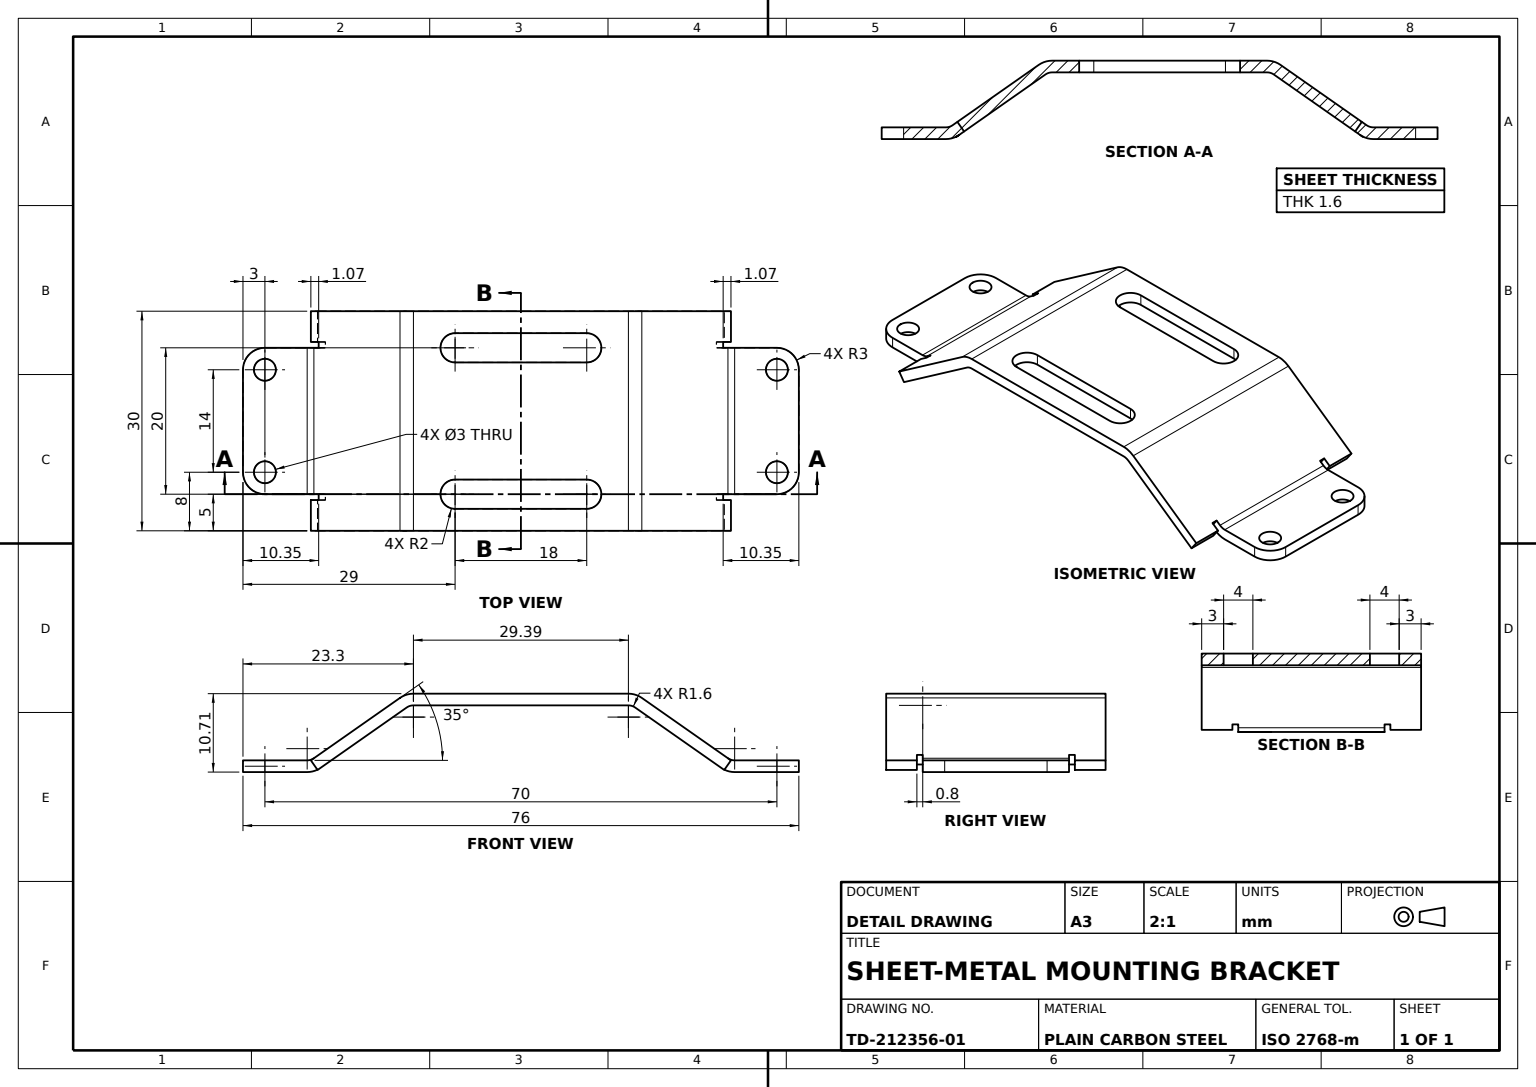
solid
v1 (29.2222,-7.511972,10)
v2 (29.2222,-7.511972,-10)
e1 v1 v2 LINE
v3 (28.304478,-7.222615,-10)
e2 v2 v3 CIRCLE(AX(P(29.2222,-5.911972,-10),D(0,0,-1),D(-1,0,0)),1.6)
v4 (28.304478,-7.222615,10)
e3 v3 v4 LINE
e4 v4 v1 CIRCLE(AX(P(29.2222,-5.911972,10),D(0,0,1),D(-1,0,0)),1.6)
face CYL(AX(P(29.2222,-5.911972,-10),D(0,0,-1),D(0,-1,0)),1.6) rev [e1 e2 e3 e4]
v5 (-27.649156,-6.763754,-10.8)
v6 (-28.717722,-7.511972,-10.8)
e5 v5 v6 LINE
v7 (-27.8,-8.822615,-10.8)
e6 v6 v7 LINE
v8 (-26.731434,-8.074397,-10.8)
e7 v8 v7 LINE
e8 v5 v8 LINE
face PLANE(AX(P(-27.649156,-6.763754,-10.8),D(0,0,1),D(0,-1,0))) [e5 e6 -e7 -e8]
v9 (-28.717722,-7.511972,10.8)
v10 (-27.649156,-6.763754,10.8)
e9 v9 v10 LINE
v11 (-26.731434,-8.074397,10.8)
e10 v10 v11 LINE
v12 (-27.8,-8.822615,10.8)
e11 v12 v11 LINE
e12 v9 v12 LINE
face PLANE(AX(P(-28.717722,-7.511972,10.8),D(0,0,-1),D(0,1,0))) [e9 e10 -e11 -e12]
v13 (-27.649156,-6.763754,10)
v14 (-28.304478,-7.222615,10)
e13 v13 v14 LINE
v15 (-27.386756,-8.533258,10)
e14 v14 v15 LINE
v16 (-26.731434,-8.074397,10)
e15 v16 v15 LINE
e16 v13 v16 LINE
face PLANE(AX(P(-27.649156,-6.763754,10),D(0,0,1),D(0,-1,0))) [e13 e14 -e15 -e16]
v17 (-29.2222,-7.511972,10)
v18 (-29.2222,-9.111972,10)
e17 v17 v18 LINE
v19 (-35,-7.511972,10)
e18 v17 v19 LINE
v20 (-35,-9.111972,10)
e19 v20 v19 LINE
e20 v18 v20 LINE
face PLANE(AX(P(-35,-9.111972,10),D(0,0,-1),D(-1,0,0))) rev [-e17 e18 -e19 -e20]
v21 (-28.304478,-7.222615,-10)
v22 (-27.386756,-8.533258,-10)
e21 v21 v22 LINE
v23 (-27.649156,-6.763754,-10)
e22 v21 v23 LINE
v24 (-26.731434,-8.074397,-10)
e23 v23 v24 LINE
e24 v22 v24 LINE
face PLANE(AX(P(-28.304478,-7.222615,-10),D(0,0,-1),D(0,1,0))) [-e21 e22 e23 -e24]
v25 (36.5,-9.111972,7)
v26 (33.5,-9.111972,7)
e25 v25 v26 CIRCLE(AX(P(35,-9.111972,7),D(0,1,0),D(-1,0,0)),1.5)
v27 (36.5,-7.511972,7)
e26 v25 v27 LINE
v28 (33.5,-7.511972,7)
e27 v27 v28 CIRCLE(AX(P(35,-7.511972,7),D(0,1,0),D(-1,0,0)),1.5)
e28 v26 v28 LINE
face CYL(AX(P(35,-9.111972,7),D(0,1,0),D(-1,0,0)),1.5) rev [-e25 e26 e27 -e28]
v29 (28.717722,-7.511972,10.8)
v30 (27.8,-8.822615,10.8)
e29 v29 v30 LINE
v31 (28.717722,-7.511972,15)
e30 v31 v29 LINE
v32 (27.8,-8.822615,15)
e31 v31 v32 LINE
e32 v32 v30 LINE
face PLANE(AX(P(28.717722,-7.511972,15),D(0.819152044,-0.573576436,0),D(0.573576436,0.819152044,0))) [-e29 -e30 e31 e32]
v33 (35,-9.111972,-10)
v34 (35,-7.511972,-10)
e33 v33 v34 LINE
v35 (29.2222,-9.111972,-10)
e34 v33 v35 LINE
e35 v2 v35 LINE
e36 v34 v2 LINE
face PLANE(AX(P(28.717722,-9.111972,-10),D(0,0,-1),D(-1,0,0))) [-e33 e34 -e35 -e36]
v36 (-16.530967,1.021287,15)
v37 (-16.530967,1.021287,-15)
e37 v36 v37 LINE
v38 (-14.695522,1.6,15)
e38 v38 v36 CIRCLE(AX(P(-14.695522,-1.6,15),D(0,0,1),D(1,0,0)),3.2)
v39 (-14.695522,1.6,-15)
e39 v38 v39 LINE
e40 v39 v37 CIRCLE(AX(P(-14.695522,-1.6,-15),D(0,0,1),D(1,0,0)),3.2)
face CYL(AX(P(-14.695522,-1.6,15),D(0,0,-1),D(-1,0,0)),3.2) [-e37 -e38 e39 e40]
e41 v10 v13 LINE
e42 v11 v16 LINE
face PLANE(AX(P(-27.649156,-6.763754,10.8),D(-0.819152044,-0.573576436,0),D(0.573576436,-0.819152044,0))) [e41 e16 -e42 -e10]
e43 v28 v27 CIRCLE(AX(P(35,-7.511972,7),D(0,1,0),D(-1,0,0)),1.5)
v40 (38,-7.511972,7)
v41 (38,-7.511972,-7)
e44 v40 v41 LINE
e45 v41 v34 CIRCLE(AX(P(35,-7.511972,-7),D(0,1,0),D(-1,0,0)),3)
v42 (35,-7.511972,10)
e46 v1 v42 LINE
e47 v42 v40 CIRCLE(AX(P(35,-7.511972,7),D(0,1,0),D(-1,0,0)),3)
v43 (33.5,-7.511972,-7)
v44 (36.5,-7.511972,-7)
e48 v43 v44 CIRCLE(AX(P(35,-7.511972,-7),D(0,1,0),D(-1,0,0)),1.5)
e49 v44 v43 CIRCLE(AX(P(35,-7.511972,-7),D(0,1,0),D(-1,0,0)),1.5)
face PLANE(AX(P(35,-7.511972,-7),D(0,1,0),D(-1,0,0))) [-e27 -e43] [e44 e45 e36 -e1 e46 e47] [-e48 -e49]
v45 (15.613244,-0.289357,-15)
v46 (16.530967,1.021287,-15)
e50 v45 v46 LINE
v47 (28.717722,-7.511972,-15)
e51 v47 v46 LINE
v48 (27.8,-8.822615,-15)
e52 v47 v48 LINE
e53 v48 v45 LINE
face PLANE(AX(P(14.695522,1.6,-15),D(0,0,-1),D(-1,0,0))) [e50 -e51 e52 e53]
v49 (27.649156,-6.763754,10)
v50 (26.731434,-8.074397,10)
e54 v49 v50 LINE
v51 (27.649156,-6.763754,10.8)
e55 v49 v51 LINE
v52 (26.731434,-8.074397,10.8)
e56 v51 v52 LINE
e57 v50 v52 LINE
face PLANE(AX(P(27.649156,-6.763754,10),D(0.819152044,-0.573576436,0),D(0.573576436,0.819152044,0))) [-e54 e55 e56 -e57]
v53 (-14.695522,0,-15)
e58 v53 v39 LINE
v54 (14.695522,1.6,-15)
e59 v54 v39 LINE
v55 (14.695522,0,-15)
e60 v54 v55 LINE
e61 v55 v53 LINE
face PLANE(AX(P(-16.530967,1.021287,-15),D(0,0,-1),D(-1,0,0))) [e58 -e59 e60 e61]
v56 (-35,-9.111972,-10)
v57 (-35,-7.511972,-10)
e62 v56 v57 LINE
v58 (-29.2222,-7.511972,-10)
e63 v57 v58 LINE
v59 (-29.2222,-9.111972,-10)
e64 v58 v59 LINE
e65 v56 v59 LINE
face PLANE(AX(P(-28.717722,-9.111972,-10),D(0,0,1),D(1,0,0))) rev [e62 e63 e64 -e65]
v60 (-27.8,-8.822615,-15)
e66 v7 v60 LINE
v61 (-15.613244,-0.289357,-15)
e67 v61 v60 LINE
v62 (-15.613244,-0.289357,15)
e68 v62 v61 LINE
v63 (-27.8,-8.822615,15)
e69 v62 v63 LINE
e70 v63 v12 LINE
e71 v15 v22 LINE
e72 v24 v8 LINE
face PLANE(AX(P(-15.2,0,15),D(0.573576436,-0.819152044,0),D(0.819152044,0.573576436,0))) [e66 -e67 -e68 e69 e70 e11 e42 e15 e71 e24 e72 e7]
v64 (29.2222,-9.111972,10)
e73 v35 v64 LINE
v65 (27.386756,-8.533258,10)
e74 v65 v64 CIRCLE(AX(P(29.2222,-5.911972,10),D(0,0,1),D(-1,0,0)),3.2)
v66 (27.386756,-8.533258,-10)
e75 v66 v65 LINE
e76 v35 v66 CIRCLE(AX(P(29.2222,-5.911972,-10),D(0,0,-1),D(-1,0,0)),3.2)
face CYL(AX(P(29.2222,-5.911972,-10),D(0,0,-1),D(0,-1,0)),3.2) [e73 -e74 -e75 -e76]
v67 (35,-9.111972,10)
v68 (38,-9.111972,7)
e77 v67 v68 CIRCLE(AX(P(35,-9.111972,7),D(0,1,0),D(-1,0,0)),3)
e78 v68 v40 LINE
e79 v67 v42 LINE
face CYL(AX(P(35,-9.111972,7),D(0,1,0),D(-1,0,0)),3) [e77 e78 -e47 -e79]
v69 (-33.5,-7.511972,-7)
v70 (-36.5,-7.511972,-7)
e80 v69 v70 CIRCLE(AX(P(-35,-7.511972,-7),D(0,-1,0),D(1,0,0)),1.5)
v71 (-33.5,-9.111972,-7)
e81 v71 v69 LINE
v72 (-36.5,-9.111972,-7)
e82 v71 v72 CIRCLE(AX(P(-35,-9.111972,-7),D(0,-1,0),D(1,0,0)),1.5)
e83 v72 v70 LINE
face CYL(AX(P(-35,-9.111972,-7),D(0,1,0),D(-1,0,0)),1.5) rev [-e80 -e81 e82 e83]
v73 (9,1.6,-8)
v74 (9,1.6,-12)
e84 v73 v74 CIRCLE(AX(P(9,1.6,-10),D(0,1,0),D(0,0,-1)),2)
v75 (-9,1.6,-8)
e85 v75 v73 LINE
v76 (-9,1.6,-12)
e86 v76 v75 CIRCLE(AX(P(-9,1.6,-10),D(0,1,0),D(0,0,-1)),2)
e87 v74 v76 LINE
v77 (14.695522,1.6,15)
e88 v77 v38 LINE
e89 v77 v54 LINE
v78 (-9,1.6,8)
v79 (-9,1.6,12)
e90 v78 v79 CIRCLE(AX(P(-9,1.6,10),D(0,1,0),D(0,0,1)),2)
v80 (9,1.6,8)
e91 v80 v78 LINE
v81 (9,1.6,12)
e92 v81 v80 CIRCLE(AX(P(9,1.6,10),D(0,1,0),D(0,0,1)),2)
e93 v79 v81 LINE
face PLANE(AX(P(-15.2,1.6,15),D(0,-1,0),D(0,0,-1))) rev [-e84 -e85 -e86 -e87] [e59 -e39 -e88 e89] [-e90 -e91 -e92 -e93]
e94 v17 v14 CIRCLE(AX(P(-29.2222,-5.911972,10),D(0,0,1),D(1,0,0)),1.6)
e95 v18 v15 CIRCLE(AX(P(-29.2222,-5.911972,10),D(0,0,1),D(1,0,0)),3.2)
face PLANE(AX(P(-29.2222,-5.911972,10),D(0,0,-1),D(-1,0,0))) rev [-e94 e17 e95 -e14]
e96 v70 v69 CIRCLE(AX(P(-35,-7.511972,-7),D(0,-1,0),D(1,0,0)),1.5)
e97 v72 v71 CIRCLE(AX(P(-35,-9.111972,-7),D(0,-1,0),D(1,0,0)),1.5)
face CYL(AX(P(-35,-9.111972,-7),D(0,1,0),D(-1,0,0)),1.5) rev [e81 -e96 -e83 e97]
e98 v4 v49 LINE
e99 v65 v50 LINE
e100 v4 v65 LINE
face PLANE(AX(P(28.304478,-7.222615,10),D(0,0,1),D(0,-1,0))) [e98 e54 -e99 -e100]
v82 (-33.5,-9.111972,7)
v83 (-33.5,-7.511972,7)
e101 v82 v83 LINE
v84 (-36.5,-7.511972,7)
e102 v84 v83 CIRCLE(AX(P(-35,-7.511972,7),D(0,-1,0),D(1,0,0)),1.5)
v85 (-36.5,-9.111972,7)
e103 v85 v84 LINE
e104 v85 v82 CIRCLE(AX(P(-35,-9.111972,7),D(0,-1,0),D(1,0,0)),1.5)
face CYL(AX(P(-35,-9.111972,7),D(0,1,0),D(-1,0,0)),1.5) rev [e101 -e102 -e103 e104]
e105 v45 v55 CIRCLE(AX(P(14.695522,-1.6,-15),D(0,0,1),D(1,0,0)),1.6)
v86 (15.613244,-0.289357,15)
e106 v86 v45 LINE
v87 (14.695522,0,15)
e107 v86 v87 CIRCLE(AX(P(14.695522,-1.6,15),D(0,0,1),D(1,0,0)),1.6)
e108 v87 v55 LINE
face CYL(AX(P(14.695522,-1.6,15),D(0,0,-1),D(-1,0,0)),1.6) rev [-e105 -e106 e107 e108]
v88 (33.5,-9.111972,-7)
e109 v88 v43 LINE
v89 (36.5,-9.111972,-7)
e110 v89 v88 CIRCLE(AX(P(35,-9.111972,-7),D(0,1,0),D(-1,0,0)),1.5)
e111 v89 v44 LINE
face CYL(AX(P(35,-9.111972,-7),D(0,1,0),D(-1,0,0)),1.5) rev [e49 -e109 -e110 e111]
v90 (-38,-7.511972,7)
e112 v19 v90 CIRCLE(AX(P(-35,-7.511972,7),D(0,-1,0),D(1,0,0)),3)
v91 (-38,-9.111972,7)
e113 v91 v90 LINE
e114 v20 v91 CIRCLE(AX(P(-35,-9.111972,7),D(0,-1,0),D(1,0,0)),3)
face CYL(AX(P(-35,-9.111972,7),D(0,1,0),D(-1,0,0)),3) [e19 e112 -e113 -e114]
e115 v53 v61 CIRCLE(AX(P(-14.695522,-1.6,-15),D(0,0,1),D(1,0,0)),1.6)
e116 v37 v61 LINE
face PLANE(AX(P(-14.695522,0,-15),D(0,0,-1),D(-1,0,0))) [-e58 e115 -e116 -e40]
e117 v32 v86 LINE
v92 (27.8,-8.822615,-10.8)
e118 v92 v48 LINE
v93 (26.731434,-8.074397,-10.8)
e119 v92 v93 LINE
v94 (26.731434,-8.074397,-10)
e120 v93 v94 LINE
e121 v94 v66 LINE
e122 v52 v30 LINE
face PLANE(AX(P(15.2,0,15),D(-0.573576436,-0.819152044,0),D(0.819152044,-0.573576436,0))) [e117 e106 -e53 -e118 e119 e120 e121 e75 e99 e57 e122 -e32]
v95 (27.649156,-6.763754,-10.8)
e123 v95 v93 LINE
v96 (27.649156,-6.763754,-10)
e124 v95 v96 LINE
e125 v96 v94 LINE
face PLANE(AX(P(27.649156,-6.763754,-10.8),D(0.819152044,-0.573576436,0),D(0.573576436,0.819152044,0))) [-e123 e124 e125 -e120]
v97 (38,-9.111972,-7)
e126 v97 v41 LINE
e127 v97 v33 CIRCLE(AX(P(35,-9.111972,-7),D(0,1,0),D(-1,0,0)),3)
face CYL(AX(P(35,-9.111972,-7),D(0,1,0),D(-1,0,0)),3) [-e45 -e126 e127 e33]
v98 (9,0,8)
e128 v98 v80 LINE
v99 (9,0,12)
e129 v99 v98 CIRCLE(AX(P(9,0,10),D(0,1,0),D(0,0,1)),2)
e130 v99 v81 LINE
face CYL(AX(P(9,0,10),D(0,1,0),D(0,0,1)),2) rev [e92 -e128 -e129 e130]
v100 (16.530967,1.021287,15)
e131 v100 v77 CIRCLE(AX(P(14.695522,-1.6,15),D(0,0,1),D(1,0,0)),3.2)
e132 v100 v46 LINE
e133 v46 v54 CIRCLE(AX(P(14.695522,-1.6,-15),D(0,0,1),D(1,0,0)),3.2)
face CYL(AX(P(14.695522,-1.6,15),D(0,0,-1),D(-1,0,0)),3.2) [-e89 -e131 e132 e133]
v101 (28.717722,-7.511972,-10.8)
e134 v101 v47 LINE
e135 v101 v92 LINE
face PLANE(AX(P(28.717722,-7.511972,15),D(0.819152044,-0.573576436,0),D(0.573576436,0.819152044,0))) [-e134 e135 e118 -e52]
e136 v62 v36 LINE
v102 (-14.695522,0,15)
e137 v102 v62 CIRCLE(AX(P(-14.695522,-1.6,15),D(0,0,1),D(1,0,0)),1.6)
e138 v38 v102 LINE
face PLANE(AX(P(-15.613244,-0.289357,15),D(0,0,1),D(1,0,0))) [e38 -e136 -e137 -e138]
e139 v100 v86 LINE
e140 v87 v77 LINE
face PLANE(AX(P(14.695522,0,15),D(0,0,1),D(1,0,0))) [-e139 e131 -e140 -e107]
e141 v26 v25 CIRCLE(AX(P(35,-9.111972,7),D(0,1,0),D(-1,0,0)),1.5)
face CYL(AX(P(35,-9.111972,7),D(0,1,0),D(-1,0,0)),1.5) rev [e28 e43 -e26 -e141]
e142 v101 v95 LINE
face PLANE(AX(P(28.717722,-7.511972,-10.8),D(0,0,1),D(1,0,0))) [e142 e123 -e119 -e135]
e143 v68 v97 LINE
face PLANE(AX(P(38,-9.111972,-7),D(1,0,0),D(0,1,0))) [-e78 e143 e126 -e44]
e144 v14 v21 LINE
v103 (-28.717722,-7.511972,15)
e145 v103 v9 LINE
e146 v36 v103 LINE
v104 (-28.717722,-7.511972,-15)
e147 v37 v104 LINE
e148 v6 v104 LINE
e149 v23 v5 LINE
face PLANE(AX(P(-16.117722,1.310643,15),D(0.573576436,-0.819152044,0),D(0.819152044,0.573576436,0))) rev [-e144 -e13 -e41 -e9 -e145 -e146 e37 e147 -e148 -e5 -e149 -e22]
v105 (9,0,-12)
e150 v105 v74 LINE
v106 (9,0,-8)
e151 v106 v105 CIRCLE(AX(P(9,0,-10),D(0,1,0),D(0,0,-1)),2)
e152 v106 v73 LINE
face CYL(AX(P(9,0,-10),D(0,1,0),D(0,0,1)),2) rev [-e150 -e151 e152 e84]
v107 (-9,0,12)
e153 v107 v79 LINE
e154 v107 v99 LINE
face PLANE(AX(P(-9,0,12),D(0,0,1),D(1,0,0))) rev [e153 e93 -e130 -e154]
e155 v1 v64 LINE
e156 v64 v67 LINE
face PLANE(AX(P(35,-9.111972,10),D(0,0,1),D(1,0,0))) [e155 e156 e79 -e46]
v108 (-9,0,-12)
e157 v108 v76 LINE
v109 (-9,0,-8)
e158 v109 v75 LINE
e159 v108 v109 CIRCLE(AX(P(-9,0,-10),D(0,1,0),D(0,0,-1)),2)
face CYL(AX(P(-9,0,-10),D(0,1,0),D(0,0,1)),2) rev [e157 e86 -e158 -e159]
e160 v21 v58 CIRCLE(AX(P(-29.2222,-5.911972,-10),D(0,0,-1),D(1,0,0)),1.6)
e161 v22 v59 CIRCLE(AX(P(-29.2222,-5.911972,-10),D(0,0,-1),D(1,0,0)),3.2)
face PLANE(AX(P(-29.2222,-5.911972,-10),D(0,0,-1),D(-1,0,0))) [-e64 -e160 e21 e161]
face PLANE(AX(P(29.2222,-5.911972,10),D(0,0,1),D(1,0,0))) [e100 e74 -e155 -e4]
e162 v31 v100 LINE
face PLANE(AX(P(-14.695522,-1.6,15),D(0,0,1),D(1,0,0))) [e139 -e117 -e31 e162]
e163 v105 v108 LINE
e164 v109 v106 LINE
e165 v87 v102 LINE
e166 v102 v53 LINE
v110 (-9,0,8)
e167 v110 v107 CIRCLE(AX(P(-9,0,10),D(0,1,0),D(0,0,1)),2)
e168 v98 v110 LINE
face PLANE(AX(P(-15.2,0,15),D(0,-1,0),D(0,0,-1))) [e163 e159 e164 e151] [-e108 e165 e166 -e61] [e167 e154 e129 e168]
e169 v110 v78 LINE
face PLANE(AX(P(-9,0,8),D(0,0,-1),D(-1,0,0))) rev [-e169 -e168 e128 e91]
v111 (-38,-9.111972,-7)
e170 v111 v56 CIRCLE(AX(P(-35,-9.111972,-7),D(0,-1,0),D(1,0,0)),3)
v112 (-38,-7.511972,-7)
e171 v111 v112 LINE
e172 v112 v57 CIRCLE(AX(P(-35,-7.511972,-7),D(0,-1,0),D(1,0,0)),3)
face CYL(AX(P(-35,-9.111972,-7),D(0,1,0),D(-1,0,0)),3) [-e170 e171 e172 -e62]
face PLANE(AX(P(-27.649156,-6.763754,-10),D(-0.819152044,-0.573576436,0),D(0.573576436,-0.819152044,0))) [-e23 e149 e8 -e72]
e173 v51 v29 LINE
face PLANE(AX(P(27.649156,-6.763754,10.8),D(0,0,-1),D(0,1,0))) [-e122 -e56 e173 e29]
face PLANE(AX(P(-9,0,-8),D(0,0,1),D(1,0,0))) rev [-e152 -e164 e158 e85]
e174 v88 v89 CIRCLE(AX(P(35,-9.111972,-7),D(0,1,0),D(-1,0,0)),1.5)
face CYL(AX(P(35,-9.111972,-7),D(0,1,0),D(-1,0,0)),1.5) rev [-e111 -e174 e109 e48]
e175 v63 v103 LINE
face PLANE(AX(P(-14.695522,1.6,15),D(0,0,1),D(1,0,0))) [e146 -e175 -e69 e136]
e176 v96 v3 LINE
e177 v3 v66 LINE
face PLANE(AX(P(27.649156,-6.763754,-10),D(0,0,-1),D(0,1,0))) [e176 e177 -e121 -e125]
face PLANE(AX(P(16.530967,1.021287,15),D(0,0,1),D(1,0,0))) [-e165 e140 e88 e138]
face PLANE(AX(P(29.2222,-5.911972,-10),D(0,0,1),D(1,0,0))) rev [-e177 -e2 e35 e76]
face PLANE(AX(P(16.117722,1.310643,15),D(-0.573576436,-0.819152044,0),D(0.819152044,-0.573576436,0))) rev [-e142 e134 e51 -e132 -e162 e30 -e173 -e55 -e98 -e3 -e176 -e124]
face CYL(AX(P(-14.695522,-1.6,15),D(0,0,-1),D(-1,0,0)),1.6) rev [-e166 e137 e68 -e115]
e178 v60 v104 LINE
face PLANE(AX(P(-27.8,-8.822615,15),D(-0.819152044,-0.573576436,0),D(0.573576436,-0.819152044,0))) [-e6 e148 -e178 -e66]
e179 v82 v85 CIRCLE(AX(P(-35,-9.111972,7),D(0,-1,0),D(1,0,0)),1.5)
e180 v18 v59 LINE
e181 v91 v111 LINE
face PLANE(AX(P(-35,-9.111972,-7),D(0,1,0),D(1,0,0))) rev [-e104 -e179] [-e180 e20 e114 e181 e170 e65] [-e97 -e82]
e182 v83 v84 CIRCLE(AX(P(-35,-7.511972,7),D(0,-1,0),D(1,0,0)),1.5)
face CYL(AX(P(-35,-9.111972,7),D(0,1,0),D(-1,0,0)),1.5) rev [-e101 e179 e103 -e182]
face PLANE(AX(P(-9,0,-12),D(0,0,-1),D(-1,0,0))) rev [e87 -e157 -e163 e150]
face CYL(AX(P(-9,0,10),D(0,1,0),D(0,0,1)),2) rev [e169 e90 -e153 -e167]
e183 v90 v112 LINE
e184 v58 v17 LINE
face PLANE(AX(P(-35,-7.511972,-7),D(0,1,0),D(1,0,0))) [e96 e80] [-e183 -e112 -e18 -e184 -e63 -e172] [e102 e182]
face PLANE(AX(P(15.613244,-0.289357,-15),D(0,0,-1),D(-1,0,0))) [-e60 -e133 -e50 e105]
face PLANE(AX(P(-14.695522,-1.6,-15),D(0,0,1),D(1,0,0))) rev [e67 e178 -e147 e116]
face CYL(AX(P(-29.2222,-5.911972,10),D(0,0,1),D(0,-1,0)),1.6) rev [e94 e144 e160 e184]
face PLANE(AX(P(-38,-9.111972,-7),D(1,0,0),D(0,1,0))) rev [e113 e183 -e171 -e181]
face CYL(AX(P(-29.2222,-5.911972,10),D(0,0,1),D(0,-1,0)),3.2) [-e161 -e71 -e95 e180]
face PLANE(AX(P(35,-9.111972,-7),D(0,1,0),D(-1,0,0))) rev [e110 e174] [e141 e25] [-e77 -e156 -e73 -e34 -e127 -e143]
face PLANE(AX(P(-27.8,-8.822615,15),D(-0.819152044,-0.573576436,0),D(0.573576436,-0.819152044,0))) [e175 e145 e12 -e70]
